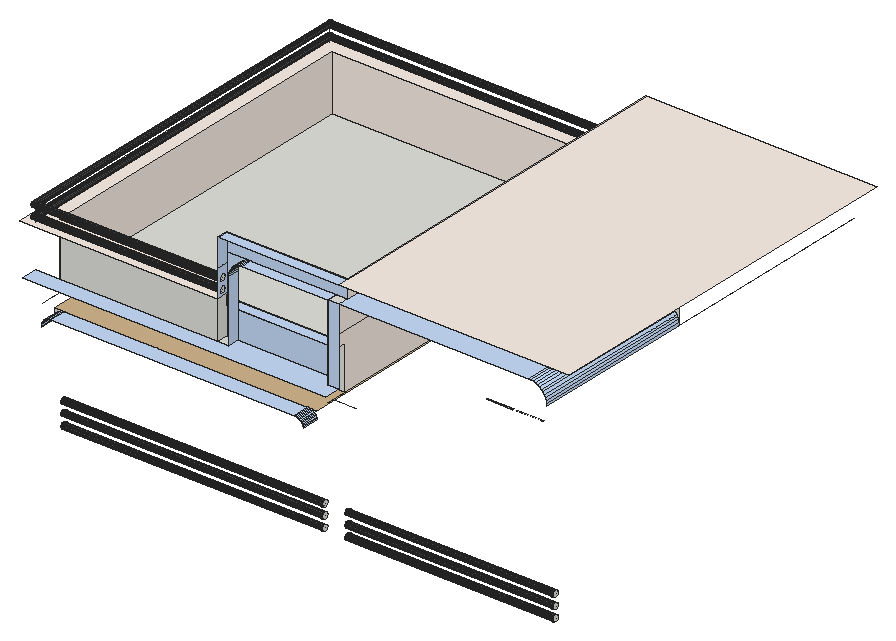
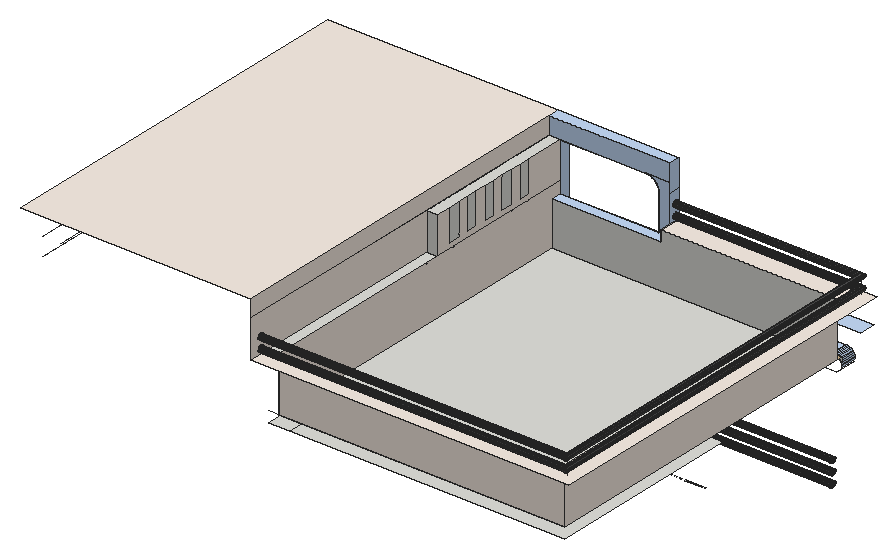
# SketchUp Ruby script. Lengths in inches.
U = 1.inch
M = Sketchup.active_model
def pt(a) = Geom::Point3d.new(a.map { |v| v * U })
def face(e, loops, mat)
  f = e.add_face(loops[0].map { |a| pt(a) })
  loops[1..].each { |l| e.add_face(l.map { |a| pt(a) }).erase! }
  f.material = f.back_material = mat if mat
  f
end
# faces: each face lists its corners as indices into pts; further lists are holes
def faces(e, pts, list, mat = nil) = list.each { |f| face(e, (f[0].is_a?(Array) ? f : [f]).map { |l| l.map { |i| pts[i] } }, mat) }
# xy, xz, yz: faces in a plane at the given z, y or x. An outline is a flat list of corners, or four numbers for a rectangle; further outlines are holes
def ring(l) = l.size == 4 ? [[l[0], l[1]], [l[2], l[1]], [l[2], l[3]], [l[0], l[3]]] : l.each_slice(2).to_a
def flat(e, list, mat, &to3) = list.each { |f| face(e, (f[0].is_a?(Array) ? f : [f]).map { |l| ring(l).map { |u, v| to3.(u, v) } }, mat) }
def xy(e, z, list, mat = nil) = flat(e, list, mat) { |x, y| [x, y, z] }
def xz(e, y, list, mat = nil) = flat(e, list, mat) { |x, z| [x, y, z] }
def yz(e, x, list, mat = nil) = flat(e, list, mat) { |y, z| [x, y, z] }
def lines(e, pts, list) = list.each { |a, b| e.add_line(pt(pts[a]), pt(pts[b])) }
# prism: a flat outline (further loops are holes) pulled along v
def prism(e, loops, v, mat = nil)
  f = face(e, loops, mat); d = Geom::Vector3d.new(v.map { |x| x * U })
  f.pushpull(f.normal.samedirection?(d) ? d.length : -d.length)
end
def box(e, o, s, mat = nil) = prism(e, [[o, [o[0] + s[0], o[1], o[2]], [o[0] + s[0], o[1] + s[1], o[2]], [o[0], o[1] + s[1], o[2]]]], [0, 0, s[2]], mat)
def at(x, y, z, deg = 0) = Geom::Transformation.translation(pt([x, y, z])) * Geom::Transformation.rotation(ORIGIN, Z_AXIS, deg.degrees)
def axes(o, x, y, z) = Geom::Transformation.new([*x, 0, *y, 0, *z, 0, *pt(o).to_a, 1])
def part(name) = M.definitions.add(name)
# library, detail: a bought-in or finely detailed component or shape, given as its bounding box
def library(name, o, s) = part(name).tap { |d| box(d.entities, o, s) }
def detail(e, o, s) = box(e.add_group.entities, o, s)
def put(e, d, t, mat = nil) = e.add_instance(d, t).tap { |i| i.material = mat if mat }
def group(e, t, mat = nil) = e.add_group.tap { |g| g.transformation = t; g.material = mat if mat }.entities
root = M.entities
M.materials.add("[0009_Linen]").color = [250, 240, 230]
M.materials.add("[0033_NavajoWhite]").color = [209, 182, 141]
M.materials.add("[0099_LightSteelBlue]").color = [198, 220, 249]
M.materials.add("[Metal Steel Textured White]").color = [84, 84, 84]
xy(root,427.88,[[43.43,263,65.05,264],[69.05,263,90.68,264],[366.6875,263,395.75,264],[399.75,263,428.8125,264]])
xy(root,428.88,[[148.81,264,198.81,266],[218.18,264,268.18,266]])
xy(root,480,[[114.29,108.66,111.1875,109.11,108.31,110.36,105.85,112.3,103.99,114.82,102.83,117.73,102.47,120.84,102.93,123.9375,104.17,126.8125,106.11,129.27,108.63,131.14,111.54,132.29,114.65,132.65,117.75,132.2,120.63,130.95,123.08,129.01,124.95,126.5,126.11,123.58,126.47,120.47,126.01,117.37,124.77,114.5,122.82,112.04,120.31,110.17,117.4,109.02],[234.29,108.66,231.1875,109.11,228.31,110.36,225.85,112.3,223.99,114.82,222.83,117.73,222.47,120.84,222.93,123.9375,224.17,126.8125,226.11,129.27,228.63,131.14,231.54,132.29,234.65,132.65,237.75,132.2,240.63,130.95,243.08,129.01,244.95,126.5,246.11,123.58,246.47,120.47,246.01,117.37,244.77,114.5,242.82,112.04,240.31,110.17,237.4,109.02],[24,264,324,480],[324,264,348,480]])
xy(root,480,[[[37.43,84,324,264],[114.29,108.66,117.4,109.02,120.31,110.17,122.82,112.04,124.77,114.5,126.01,117.37,126.47,120.47,126.11,123.58,124.95,126.5,123.08,129.01,120.63,130.95,117.75,132.2,114.65,132.65,111.54,132.29,108.63,131.14,106.11,129.27,104.17,126.8125,102.93,123.9375,102.47,120.84,102.83,117.73,103.99,114.82,105.85,112.3,108.31,110.36,111.1875,109.11],[234.29,108.66,237.4,109.02,240.31,110.17,242.82,112.04,244.77,114.5,246.01,117.37,246.47,120.47,246.11,123.58,244.95,126.5,243.08,129.01,240.63,130.95,237.75,132.2,234.65,132.65,231.54,132.29,228.63,131.14,226.11,129.27,224.17,126.8125,222.93,123.9375,222.47,120.84,222.83,117.73,223.99,114.82,225.85,112.3,228.31,110.36,231.1875,109.11]]],"[0033_NavajoWhite]")
xy(root,480,[[48.16,66,314.66,84]],"[0099_LightSteelBlue]")
xy(root,492,[[24,108,336,480]])
xy(root,510,[[216,84,228,96]])
xy(root,510,[[17.11,66,348,66,348,84,336,84,336,96,228,96,228,84,17.11,84]],"[0099_LightSteelBlue]")
xy(root,540,[[216,96,336,108]],"[0099_LightSteelBlue]")
xy(root,552,[[336,264,348,480]])
xy(root,552,[[0,84,216,84,216,108,24,108,24,480,348,480,348,504,0,504]],"[0009_Linen]")
xy(root,582,[[215.9375,84,216,96]])
xy(root,592.85,[[336,84,348,96],[336,96,348,264],[442.72,124.07,439.67,124.77,436.9,126.23,434.6,128.36,432.93,131.01,432.01,134.01,431.89,137.14,432.59,140.19,434.05,142.96,436.18,145.26,438.83,146.93,441.83,147.85,444.96,147.97,448.01,147.27,450.78,145.81,453.08,143.68,454.75,141.03,455.67,138.03,455.79,134.9,455.09,131.85,453.63,129.08,451.5,126.78,448.85,125.11,445.85,124.19]])
xy(root,592.85,[[242.86,84,336,96],[[348,84,556.05,264],[442.72,124.07,445.85,124.19,448.85,125.11,451.5,126.78,453.63,129.08,455.09,131.85,455.79,134.9,455.67,138.03,454.75,141.03,453.08,143.68,450.78,145.81,448.01,147.27,444.96,147.97,441.83,147.85,438.83,146.93,436.18,145.26,434.05,142.96,432.59,140.19,431.89,137.14,432.01,134.01,432.93,131.01,434.6,128.36,436.9,126.23,439.67,124.77]]],"[0099_LightSteelBlue]")
xy(root,612,[[348,84,600,504]],"[0009_Linen]")
xy(root,612,[[216,84,348,96]],"[0099_LightSteelBlue]")
xz(root,84,[[37.43,469.26,37.43,480,48.16,480,46.76,479.91,45.38,479.63,44.05,479.18,42.79,478.5625,41.625,477.78,40.57,476.85,39.64,475.8,38.86,474.63,38.24,473.37,37.79,472.04,37.52,470.66],[215.9375,582,216,592.85]])
xz(root,84,[[336,510,348,592.85]],"[0099_LightSteelBlue]")
xz(root,96,[[216,510,228,540],[215.9375,582,216,592.85]])
xz(root,96,[[228,510,336,540],[216,540,216,592.85,242.86,592.85,240.92,592.72,239.01,592.35,237.17,591.72,235.43,590.86,233.8125,589.78,232.35,588.5,231.07,587.04,229.99,585.42,229.13,583.68,228.51,581.84,228.13,579.93,228,577.99,228,540],[216,592.85,348,612]],"[0099_LightSteelBlue]")
xz(root,108,[[24,492,24,552,216,552,216,540,336,540,336,492]])
xz(root,264,[[336,552,348,592.85],[576,572.9,576,592.85,556.05,592.85,558.65,592.68,561.21,592.17,563.68,591.33,566.02,590.18,568.19,588.73,570.16,587.01,571.875,585.05,573.33,582.875,574.48,580.53,575.32,578.0625,575.83,575.5]])
xz(root,480,[[24,492,336,552]],"[0009_Linen]")
yz(root,24,[[108,492,480,552]],"[0009_Linen]")
yz(root,216,[[84,510,96,552],[96,540,108,552],[90,555,90.78,555.1,91.5,555.4,92.12,555.88,92.6,556.5,92.9,557.22,93,558,92.9,558.78,92.6,559.5,92.12,560.12,91.5,560.6,90.78,560.9,90,561,89.22,560.9,88.5,560.6,87.88,560.12,87.4,559.5,87.1,558.78,87,558,87.1,557.22,87.4,556.5,87.88,555.88,88.5,555.4,89.22,555.1],[90,567,90.78,567.1,91.5,567.4,92.12,567.88,92.6,568.5,92.9,569.22,93,570,92.9,570.78,92.6,571.5,92.12,572.12,91.5,572.6,90.78,572.9,90,573,89.22,572.9,88.5,572.6,87.88,572.12,87.4,571.5,87.1,570.78,87,570,87.1,569.22,87.4,568.5,87.88,567.88,88.5,567.4,89.22,567.1]])
yz(root,216,[[[84,552,96,582],[90,567,90.78,567.1,91.5,567.4,92.12,567.88,92.6,568.5,92.9,569.22,93,570,92.9,570.78,92.6,571.5,92.12,572.12,91.5,572.6,90.78,572.9,90,573,89.22,572.9,88.5,572.6,87.88,572.12,87.4,571.5,87.1,570.78,87,570,87.1,569.22,87.4,568.5,87.88,567.88,88.5,567.4,89.22,567.1],[90,555,90.78,555.1,91.5,555.4,92.12,555.88,92.6,556.5,92.9,557.22,93,558,92.9,558.78,92.6,559.5,92.12,560.12,91.5,560.6,90.78,560.9,90,561,89.22,560.9,88.5,560.6,87.88,560.12,87.4,559.5,87.1,558.78,87,558,87.1,557.22,87.4,556.5,87.88,555.88,88.5,555.4,89.22,555.1]],[84,582,96,612]],"[0099_LightSteelBlue]")
yz(root,228,[[84,510,96,577.99]],"[0099_LightSteelBlue]")
yz(root,324,[[96,357,96.78,357.1,97.5,357.4,98.12,357.88,98.6,358.5,98.9,359.22,99,360,98.9,360.78,98.6,361.5,98.12,362.12,97.5,362.6,96.78,362.9,96,363,95.22,362.9,94.5,362.6,93.88,362.12,93.4,361.5,93.1,360.78,93,360,93.1,359.22,93.4,358.5,93.88,357.88,94.5,357.4,95.22,357.1],[96,369,96.78,369.1,97.5,369.4,98.12,369.88,98.6,370.5,98.9,371.22,99,372,98.9,372.78,98.6,373.5,98.12,374.12,97.5,374.6,96.78,374.9,96,375,95.22,374.9,94.5,374.6,93.88,374.12,93.4,373.5,93.1,372.78,93,372,93.1,371.22,93.4,370.5,93.88,369.88,94.5,369.4,95.22,369.1],[96,381,96.78,381.1,97.5,381.4,98.12,381.88,98.6,382.5,98.9,383.22,99,384,98.9,384.78,98.6,385.5,98.12,386.12,97.5,386.6,96.78,386.9,96,387,95.22,386.9,94.5,386.6,93.88,386.12,93.4,385.5,93.1,384.78,93,384,93.1,383.22,93.4,382.5,93.88,381.88,94.5,381.4,95.22,381.1]])
yz(root,336,[[139.26,558.48,151.57,592.85],[163.26,558.48,175.57,592.85],[187.26,558.48,199.57,592.85],[211.26,558.48,223.57,592.85],[235.26,558.48,247.57,592.85]])
yz(root,336,[[108,492,108,540,96,540,96,552,480,552,480,492],[96,552,96,592.85,139.26,592.85,139.26,558.48,151.57,558.48,151.57,592.85,163.26,592.85,163.26,558.48,175.57,558.48,175.57,592.85,187.26,592.85,187.26,558.48,199.57,558.48,199.57,592.85,211.26,592.85,211.26,558.48,223.57,558.48,223.57,592.85,235.26,592.85,235.26,558.48,247.57,558.48,247.57,592.85,264,592.85,264,552]],"[0009_Linen]")
yz(root,336,[[84,510,96,592.85]],"[0099_LightSteelBlue]")
yz(root,348,[[[264,552,504,592.85],[492,567,492.78,567.1,493.5,567.4,494.12,567.88,494.6,568.5,494.9,569.22,495,570,494.9,570.78,494.6,571.5,494.12,572.12,493.5,572.6,492.78,572.9,492,573,491.22,572.9,490.5,572.6,489.88,572.12,489.4,571.5,489.1,570.78,489,570,489.1,569.22,489.4,568.5,489.88,567.88,490.5,567.4,491.22,567.1],[492,555,492.78,555.1,493.5,555.4,494.12,555.88,494.6,556.5,494.9,557.22,495,558,494.9,558.78,494.6,559.5,494.12,560.12,493.5,560.6,492.78,560.9,492,561,491.22,560.9,490.5,560.6,489.88,560.12,489.4,559.5,489.1,558.78,489,558,489.1,557.22,489.4,556.5,489.88,555.88,490.5,555.4,491.22,555.1]],[96,592.85,504,612]],"[0009_Linen]")
yz(root,576,[[96,357,96.78,357.1,97.5,357.4,98.12,357.88,98.6,358.5,98.9,359.22,99,360,98.9,360.78,98.6,361.5,98.12,362.12,97.5,362.6,96.78,362.9,96,363,95.22,362.9,94.5,362.6,93.88,362.12,93.4,361.5,93.1,360.78,93,360,93.1,359.22,93.4,358.5,93.88,357.88,94.5,357.4,95.22,357.1],[96,369,96.78,369.1,97.5,369.4,98.12,369.88,98.6,370.5,98.9,371.22,99,372,98.9,372.78,98.6,373.5,98.12,374.12,97.5,374.6,96.78,374.9,96,375,95.22,374.9,94.5,374.6,93.88,374.12,93.4,373.5,93.1,372.78,93,372,93.1,371.22,93.4,370.5,93.88,369.88,94.5,369.4,95.22,369.1],[96,381,96.78,381.1,97.5,381.4,98.12,381.88,98.6,382.5,98.9,383.22,99,384,98.9,384.78,98.6,385.5,98.12,386.12,97.5,386.6,96.78,386.9,96,387,95.22,386.9,94.5,386.6,93.88,386.12,93.4,385.5,93.1,384.78,93,384,93.1,383.22,93.4,382.5,93.88,381.88,94.5,381.4,95.22,381.1]])
p = [[324,96,357],[324,95.22,357.1],[37.43,95.22,357.1],[37.43,96,357],[576,96,357],[576,95.22,357.1],
  [348,95.22,357.1],[348,96,357],[324,96.78,357.1],[37.43,96.78,357.1],[576,96.78,357.1],[348,96.78,357.1],
  [324,94.5,357.4],[37.43,94.5,357.4],[576,94.5,357.4],[348,94.5,357.4],[324,97.5,357.4],[37.43,97.5,357.4],
  [576,97.5,357.4],[348,97.5,357.4],[324,93.88,357.88],[37.43,93.88,357.88],[576,93.88,357.88],[348,93.88,357.88],
  [324,98.12,357.88],[37.43,98.12,357.88],[576,98.12,357.88],[348,98.12,357.88],[324,93.4,358.5],[37.43,93.4,358.5],
  [576,93.4,358.5],[348,93.4,358.5],[324,98.6,358.5],[37.43,98.6,358.5],[576,98.6,358.5],[348,98.6,358.5],
  [324,93.1,359.22],[37.43,93.1,359.22],[576,93.1,359.22],[348,93.1,359.22],[324,98.9,359.22],[37.43,98.9,359.22],
  [576,98.9,359.22],[348,98.9,359.22],[324,93,360],[37.43,93,360],[576,93,360],[348,93,360],
  [324,99,360],[37.43,99,360],[576,99,360],[348,99,360],[324,93.1,360.78],[37.43,93.1,360.78],
  [576,93.1,360.78],[348,93.1,360.78],[324,98.9,360.78],[37.43,98.9,360.78],[576,98.9,360.78],[348,98.9,360.78],
  [324,93.4,361.5],[37.43,93.4,361.5],[576,93.4,361.5],[348,93.4,361.5],[324,98.6,361.5],[37.43,98.6,361.5],
  [576,98.6,361.5],[348,98.6,361.5],[324,93.88,362.12],[37.43,93.88,362.12],[576,93.88,362.12],[348,93.88,362.12],
  [324,98.12,362.12],[37.43,98.12,362.12],[576,98.12,362.12],[348,98.12,362.12],[324,94.5,362.6],[37.43,94.5,362.6],
  [576,94.5,362.6],[348,94.5,362.6],[324,97.5,362.6],[37.43,97.5,362.6],[576,97.5,362.6],[348,97.5,362.6],
  [324,95.22,362.9],[37.43,95.22,362.9],[576,95.22,362.9],[348,95.22,362.9],[324,96.78,362.9],[37.43,96.78,362.9],
  [576,96.78,362.9],[348,96.78,362.9],[324,96,363],[37.43,96,363],[576,96,363],[348,96,363],
  [324,96,369],[324,95.22,369.1],[37.43,95.22,369.1],[37.43,96,369],[576,96,369],[576,95.22,369.1],
  [348,95.22,369.1],[348,96,369],[324,96.78,369.1],[37.43,96.78,369.1],[576,96.78,369.1],[348,96.78,369.1],
  [324,94.5,369.4],[37.43,94.5,369.4],[576,94.5,369.4],[348,94.5,369.4],[324,97.5,369.4],[37.43,97.5,369.4],
  [576,97.5,369.4],[348,97.5,369.4],[324,93.88,369.88],[37.43,93.88,369.88],[576,93.88,369.88],[348,93.88,369.88],
  [324,98.12,369.88],[37.43,98.12,369.88],[576,98.12,369.88],[348,98.12,369.88],[324,93.4,370.5],[37.43,93.4,370.5],
  [576,93.4,370.5],[348,93.4,370.5],[324,98.6,370.5],[37.43,98.6,370.5],[576,98.6,370.5],[348,98.6,370.5],
  [324,93.1,371.22],[37.43,93.1,371.22],[576,93.1,371.22],[348,93.1,371.22],[324,98.9,371.22],[37.43,98.9,371.22],
  [576,98.9,371.22],[348,98.9,371.22],[324,93,372],[37.43,93,372],[576,93,372],[348,93,372],
  [324,99,372],[37.43,99,372],[576,99,372],[348,99,372],[324,93.1,372.78],[37.43,93.1,372.78],
  [576,93.1,372.78],[348,93.1,372.78],[324,98.9,372.78],[37.43,98.9,372.78],[576,98.9,372.78],[348,98.9,372.78],
  [324,93.4,373.5],[37.43,93.4,373.5],[576,93.4,373.5],[348,93.4,373.5],[324,98.6,373.5],[37.43,98.6,373.5],
  [576,98.6,373.5],[348,98.6,373.5],[324,93.88,374.12],[37.43,93.88,374.12],[576,93.88,374.12],[348,93.88,374.12],
  [324,98.12,374.12],[37.43,98.12,374.12],[576,98.12,374.12],[348,98.12,374.12],[324,94.5,374.6],[37.43,94.5,374.6],
  [576,94.5,374.6],[348,94.5,374.6],[324,97.5,374.6],[37.43,97.5,374.6],[576,97.5,374.6],[348,97.5,374.6],
  [324,95.22,374.9],[37.43,95.22,374.9],[576,95.22,374.9],[348,95.22,374.9],[324,96.78,374.9],[37.43,96.78,374.9],
  [576,96.78,374.9],[348,96.78,374.9],[324,96,375],[37.43,96,375],[576,96,375],[348,96,375],
  [324,96,381],[324,95.22,381.1],[37.43,95.22,381.1],[37.43,96,381],[576,96,381],[576,95.22,381.1],
  [348,95.22,381.1],[348,96,381],[324,96.78,381.1],[37.43,96.78,381.1],[576,96.78,381.1],[348,96.78,381.1],
  [324,94.5,381.4],[37.43,94.5,381.4],[576,94.5,381.4],[348,94.5,381.4],[324,97.5,381.4],[37.43,97.5,381.4],
  [576,97.5,381.4],[348,97.5,381.4],[324,93.88,381.88],[37.43,93.88,381.88],[576,93.88,381.88],[348,93.88,381.88],
  [324,98.12,381.88],[37.43,98.12,381.88],[576,98.12,381.88],[348,98.12,381.88],[324,93.4,382.5],[37.43,93.4,382.5],
  [576,93.4,382.5],[348,93.4,382.5],[324,98.6,382.5],[37.43,98.6,382.5],[576,98.6,382.5],[348,98.6,382.5],
  [324,93.1,383.22],[37.43,93.1,383.22],[576,93.1,383.22],[348,93.1,383.22],[324,98.9,383.22],[37.43,98.9,383.22],
  [576,98.9,383.22],[348,98.9,383.22],[324,93,384],[37.43,93,384],[576,93,384],[348,93,384],
  [324,99,384],[37.43,99,384],[576,99,384],[348,99,384],[324,93.1,384.78],[37.43,93.1,384.78],
  [576,93.1,384.78],[348,93.1,384.78],[324,98.9,384.78],[37.43,98.9,384.78],[576,98.9,384.78],[348,98.9,384.78],
  [324,93.4,385.5],[37.43,93.4,385.5],[576,93.4,385.5],[348,93.4,385.5],[324,98.6,385.5],[37.43,98.6,385.5],
  [576,98.6,385.5],[348,98.6,385.5],[324,93.88,386.12],[37.43,93.88,386.12],[576,93.88,386.12],[348,93.88,386.12],
  [324,98.12,386.12],[37.43,98.12,386.12],[576,98.12,386.12],[348,98.12,386.12],[324,94.5,386.6],[37.43,94.5,386.6],
  [576,94.5,386.6],[348,94.5,386.6],[324,97.5,386.6],[37.43,97.5,386.6],[576,97.5,386.6],[348,97.5,386.6],
  [324,95.22,386.9],[37.43,95.22,386.9],[576,95.22,386.9],[348,95.22,386.9],[324,96.78,386.9],[37.43,96.78,386.9],
  [576,96.78,386.9],[348,96.78,386.9],[324,96,387],[37.43,96,387],[576,96,387],[348,96,387],
  [37.43,84,469.26],[37.52,84,470.66],[37.52,66,470.66],[37.43,66,469.26],[37.79,84,472.04],[37.79,66,472.04],
  [323.92,84,471.88],[324,84,470.66],[324,66,470.66],[323.92,66,471.88],[323.68,84,473.08],[323.68,66,473.08],
  [38.24,84,473.37],[38.24,66,473.37],[323.29,84,474.24],[323.29,66,474.24],[38.86,84,474.63],[38.86,66,474.63],
  [322.75,84,475.33],[322.75,66,475.33],[39.64,84,475.8],[39.64,66,475.8],[322.07,84,476.35],[322.07,66,476.35],
  [40.57,84,476.85],[40.57,66,476.85],[321.27,84,477.27],[321.27,66,477.27],[41.625,84,477.78],[41.625,66,477.78],
  [320.35,84,478.07],[320.35,66,478.07],[42.79,84,478.5625],[42.79,66,478.5625],[319.33,84,478.75],[319.33,66,478.75],
  [44.05,84,479.18],[44.05,66,479.18],[318.24,84,479.29],[318.24,66,479.29],[45.38,84,479.63],[45.38,66,479.63],
  [317.08,84,479.68],[317.08,66,479.68],[46.76,84,479.91],[46.76,66,479.91],[315.88,84,479.92],[315.88,66,479.92],
  [48.16,84,480],[48.16,66,480],[314.66,84,480],[314.66,66,480],[216,90,555],[216,89.22,555.1],
  [11.22,89.22,555.1],[12,90,555],[11.22,492.78,555.1],[12,492,555],[216,90.78,555.1],[12.78,90.78,555.1],
  [12.78,491.22,555.1],[348,492,555],[348,491.22,555.1],[348,492.78,555.1],[216,88.5,555.4],[10.5,88.5,555.4],
  [10.5,493.5,555.4],[216,91.5,555.4],[13.5,91.5,555.4],[13.5,490.5,555.4],[348,490.5,555.4],[348,493.5,555.4],
  [216,87.88,555.88],[9.88,87.88,555.88],[9.88,494.12,555.88],[216,92.12,555.88],[14.12,92.12,555.88],[14.12,489.88,555.88],
  [348,489.88,555.88],[348,494.12,555.88],[216,87.4,556.5],[9.4,87.4,556.5],[9.4,494.6,556.5],[216,92.6,556.5],
  [14.6,92.6,556.5],[14.6,489.4,556.5],[348,489.4,556.5],[348,494.6,556.5],[216,87.1,557.22],[9.1,87.1,557.22],
  [9.1,494.9,557.22],[216,92.9,557.22],[14.9,92.9,557.22],[14.9,489.1,557.22],[348,489.1,557.22],[348,494.9,557.22],
  [216,87,558],[9,87,558],[9,495,558],[216,93,558],[15,93,558],[15,489,558],
  [348,489,558],[348,495,558],[216,87.1,558.78],[9.1,87.1,558.78],[9.1,494.9,558.78],[216,92.9,558.78],
  [14.9,92.9,558.78],[14.9,489.1,558.78],[348,489.1,558.78],[348,494.9,558.78],[216,87.4,559.5],[9.4,87.4,559.5],
  [9.4,494.6,559.5],[216,92.6,559.5],[14.6,92.6,559.5],[14.6,489.4,559.5],[348,489.4,559.5],[348,494.6,559.5],
  [216,87.88,560.12],[9.88,87.88,560.12],[9.88,494.12,560.12],[216,92.12,560.12],[14.12,92.12,560.12],[14.12,489.88,560.12],
  [348,489.88,560.12],[348,494.12,560.12],[216,88.5,560.6],[10.5,88.5,560.6],[10.5,493.5,560.6],[216,91.5,560.6],
  [13.5,91.5,560.6],[13.5,490.5,560.6],[348,490.5,560.6],[348,493.5,560.6],[216,89.22,560.9],[11.22,89.22,560.9],
  [11.22,492.78,560.9],[216,90.78,560.9],[12.78,90.78,560.9],[12.78,491.22,560.9],[348,491.22,560.9],[348,492.78,560.9],
  [216,90,561],[12,90,561],[12,492,561],[348,492,561],[216,90,567],[216,89.22,567.1],
  [11.22,89.22,567.1],[12,90,567],[11.22,492.78,567.1],[12,492,567],[216,90.78,567.1],[12.78,90.78,567.1],
  [12.78,491.22,567.1],[348,492,567],[348,491.22,567.1],[348,492.78,567.1],[216,88.5,567.4],[10.5,88.5,567.4],
  [10.5,493.5,567.4],[216,91.5,567.4],[13.5,91.5,567.4],[13.5,490.5,567.4],[348,490.5,567.4],[348,493.5,567.4],
  [216,87.88,567.88],[9.88,87.88,567.88],[9.88,494.12,567.88],[216,92.12,567.88],[14.12,92.12,567.88],[14.12,489.88,567.88],
  [348,489.88,567.88],[348,494.12,567.88],[216,87.4,568.5],[9.4,87.4,568.5],[9.4,494.6,568.5],[216,92.6,568.5],
  [14.6,92.6,568.5],[14.6,489.4,568.5],[348,489.4,568.5],[348,494.6,568.5],[216,87.1,569.22],[9.1,87.1,569.22],
  [9.1,494.9,569.22],[216,92.9,569.22],[14.9,92.9,569.22],[14.9,489.1,569.22],[348,489.1,569.22],[348,494.9,569.22],
  [216,87,570],[9,87,570],[9,495,570],[216,93,570],[15,93,570],[15,489,570],
  [348,489,570],[348,495,570],[216,87.1,570.78],[9.1,87.1,570.78],[9.1,494.9,570.78],[216,92.9,570.78],
  [14.9,92.9,570.78],[14.9,489.1,570.78],[348,489.1,570.78],[348,494.9,570.78],[216,87.4,571.5],[9.4,87.4,571.5],
  [9.4,494.6,571.5],[216,92.6,571.5],[14.6,92.6,571.5],[14.6,489.4,571.5],[348,489.4,571.5],[348,494.6,571.5],
  [216,87.88,572.12],[9.88,87.88,572.12],[9.88,494.12,572.12],[216,92.12,572.12],[14.12,92.12,572.12],[14.12,489.88,572.12],
  [348,489.88,572.12],[348,494.12,572.12],[216,88.5,572.6],[10.5,88.5,572.6],[10.5,493.5,572.6],[216,91.5,572.6],
  [13.5,91.5,572.6],[13.5,490.5,572.6],[348,490.5,572.6],[348,493.5,572.6],[216,89.22,572.9],[11.22,89.22,572.9],
  [11.22,492.78,572.9],[216,90.78,572.9],[12.78,90.78,572.9],[12.78,491.22,572.9],[348,491.22,572.9],[348,492.78,572.9],
  [575.83,84,575.5],[575.83,264,575.5],[576,264,572.9],[576,84,572.9],[216,90,573],[12,90,573],
  [12,492,573],[348,492,573],[575.32,84,578.0625],[575.32,264,578.0625],[228.13,84,579.93],[228,84,577.99],
  [228,96,577.99],[228.13,96,579.93],[574.48,84,580.53],[574.48,264,580.53],[228.51,84,581.84],[228.51,96,581.84],
  [573.33,84,582.875],[573.33,264,582.875],[229.13,84,583.68],[229.13,96,583.68],[571.875,84,585.05],[571.875,264,585.05],
  [229.99,84,585.42],[229.99,96,585.42],[570.16,84,587.01],[570.16,264,587.01],[231.07,84,587.04],[231.07,96,587.04],
  [232.35,84,588.5],[232.35,96,588.5],[568.19,84,588.73],[568.19,264,588.73],[233.8125,84,589.78],[233.8125,96,589.78],
  [566.02,84,590.18],[566.02,264,590.18],[235.43,84,590.86],[235.43,96,590.86],[563.68,84,591.33],[563.68,264,591.33],
  [237.17,84,591.72],[237.17,96,591.72],[561.21,84,592.17],[561.21,264,592.17],[239.01,84,592.35],[239.01,96,592.35],
  [558.65,84,592.68],[558.65,264,592.68],[240.92,84,592.72],[240.92,96,592.72],[242.86,84,592.85],[242.86,96,592.85],
  [556.05,84,592.85],[556.05,264,592.85],[324,108,480],[348,108,480],[336,108,492],[336,84,492],
  [336,480,492],[348,480,492],[336,480,549.9375],[348,480,549.9375],[24,108,480],[37.43,108,480],
  [24,84,480],[324,84,480],[324,66,480],[576,264,592.85],[576,504,592.85],[556.05,504,592.85],
  [576,504,572.9],[576,96,384],[348,96,384],[324,96,384],[37.43,96,384],[37.43,96,372],
  [324,96,372],[37.43,96,360],[324,96,360],[348,96,372],[576,96,372],[348,96,360],
  [576,96,360],[12,90,552],[12,90,570],[216,90,570],[12,492,570],[12,492,552],
  [348,492,570],[12,90,558],[216,90,558],[12,492,558],[348,492,558]]
faces(root,p,[[0,1,2,3],[4,5,6,7],[8,0,3,9],[10,4,7,11],[1,12,13,2],[5,14,15,6],[16,8,9,17],[18,10,11,19],
  [12,20,21,13],[14,22,23,15],[24,16,17,25],[26,18,19,27],[20,28,29,21],[22,30,31,23],[32,24,25,33],[34,26,27,35],
  [28,36,37,29],[30,38,39,31],[40,32,33,41],[42,34,35,43],[36,44,45,37],[38,46,47,39],[48,40,41,49],[50,42,43,51],
  [44,52,53,45],[46,54,55,47],[56,48,49,57],[58,50,51,59],[52,60,61,53],[54,62,63,55],[64,56,57,65],[66,58,59,67],
  [60,68,69,61],[62,70,71,63],[72,64,65,73],[74,66,67,75],[68,76,77,69],[70,78,79,71],[80,72,73,81],[82,74,75,83],
  [76,84,85,77],[78,86,87,79],[88,80,81,89],[90,82,83,91],[84,92,93,85],[86,94,95,87],[92,88,89,93],[94,90,91,95],
  [96,97,98,99],[100,101,102,103],[104,96,99,105],[106,100,103,107],[97,108,109,98],[101,110,111,102],[112,104,105,113],[114,106,107,115],
  [108,116,117,109],[110,118,119,111],[120,112,113,121],[122,114,115,123],[116,124,125,117],[118,126,127,119],[128,120,121,129],[130,122,123,131],
  [124,132,133,125],[126,134,135,127],[136,128,129,137],[138,130,131,139],[132,140,141,133],[134,142,143,135],[144,136,137,145],[146,138,139,147],
  [140,148,149,141],[142,150,151,143],[152,144,145,153],[154,146,147,155],[148,156,157,149],[150,158,159,151],[160,152,153,161],[162,154,155,163],
  [156,164,165,157],[158,166,167,159],[168,160,161,169],[170,162,163,171],[164,172,173,165],[166,174,175,167],[176,168,169,177],[178,170,171,179],
  [172,180,181,173],[174,182,183,175],[184,176,177,185],[186,178,179,187],[180,188,189,181],[182,190,191,183],[188,184,185,189],[190,186,187,191],
  [192,193,194,195],[196,197,198,199],[200,192,195,201],[202,196,199,203],[193,204,205,194],[197,206,207,198],[208,200,201,209],[210,202,203,211],
  [204,212,213,205],[206,214,215,207],[216,208,209,217],[218,210,211,219],[212,220,221,213],[214,222,223,215],[224,216,217,225],[226,218,219,227],
  [220,228,229,221],[222,230,231,223],[232,224,225,233],[234,226,227,235],[228,236,237,229],[230,238,239,231],[240,232,233,241],[242,234,235,243],
  [236,244,245,237],[238,246,247,239],[248,240,241,249],[250,242,243,251],[244,252,253,245],[246,254,255,247],[256,248,249,257],[258,250,251,259],
  [252,260,261,253],[254,262,263,255],[264,256,257,265],[266,258,259,267],[260,268,269,261],[262,270,271,263],[272,264,265,273],[274,266,267,275],
  [268,276,277,269],[270,278,279,271],[280,272,273,281],[282,274,275,283],[276,284,285,277],[278,286,287,279],[284,280,281,285],[286,282,283,287],
  [340,341,342,343],[343,342,344,345],[346,340,343,347],[347,343,345,348],[348,345,349,350],[345,344,351,349],[341,352,353,342],[342,353,354,344],
  [355,346,347,356],[356,347,348,357],[357,348,350,358],[344,354,359,351],[352,360,361,353],[353,361,362,354],[363,355,356,364],[364,356,357,365],
  [365,357,358,366],[354,362,367,359],[360,368,369,361],[361,369,370,362],[371,363,364,372],[372,364,365,373],[373,365,366,374],[362,370,375,367],
  [368,376,377,369],[369,377,378,370],[379,371,372,380],[380,372,373,381],[381,373,374,382],[370,378,383,375],[376,384,385,377],[377,385,386,378],
  [387,379,380,388],[388,380,381,389],[389,381,382,390],[378,386,391,383],[384,392,393,385],[385,393,394,386],[395,387,388,396],[396,388,389,397],
  [397,389,390,398],[386,394,399,391],[392,400,401,393],[393,401,402,394],[403,395,396,404],[404,396,397,405],[405,397,398,406],[394,402,407,399],
  [400,408,409,401],[401,409,410,402],[411,403,404,412],[412,404,405,413],[413,405,406,414],[402,410,415,407],[408,416,417,409],[409,417,418,410],
  [419,411,412,420],[420,412,413,421],[421,413,414,422],[410,418,423,415],[416,424,425,417],[417,425,426,418],[427,419,420,428],[428,420,421,429],
  [429,421,422,430],[418,426,431,423],[424,432,433,425],[425,433,434,426],[432,427,428,433],[433,428,429,434],[434,429,430,435],[426,434,435,431],
  [436,437,438,439],[439,438,440,441],[442,436,439,443],[443,439,441,444],[444,441,445,446],[441,440,447,445],[437,448,449,438],[438,449,450,440],
  [451,442,443,452],[452,443,444,453],[453,444,446,454],[440,450,455,447],[448,456,457,449],[449,457,458,450],[459,451,452,460],[460,452,453,461],
  [461,453,454,462],[450,458,463,455],[456,464,465,457],[457,465,466,458],[467,459,460,468],[468,460,461,469],[469,461,462,470],[458,466,471,463],
  [464,472,473,465],[465,473,474,466],[475,467,468,476],[476,468,469,477],[477,469,470,478],[466,474,479,471],[472,480,481,473],[473,481,482,474],
  [483,475,476,484],[484,476,477,485],[485,477,478,486],[474,482,487,479],[480,488,489,481],[481,489,490,482],[491,483,484,492],[492,484,485,493],
  [493,485,486,494],[482,490,495,487],[488,496,497,489],[489,497,498,490],[499,491,492,500],[500,492,493,501],[501,493,494,502],[490,498,503,495],
  [496,504,505,497],[497,505,506,498],[507,499,500,508],[508,500,501,509],[509,501,502,510],[498,506,511,503],[504,512,513,505],[505,513,514,506],
  [515,507,508,516],[516,508,509,517],[517,509,510,518],[506,514,519,511],[512,520,521,513],[513,521,522,514],[523,515,516,524],[524,516,517,525],
  [525,517,518,526],[514,522,527,519],[520,532,533,521],[521,533,534,522],[532,523,524,533],[533,524,525,534],[534,525,526,535],[522,534,535,527]],"[Metal Steel Textured White]")
faces(root,p,[[288,289,290,291],[289,292,293,290],[294,295,296,297],[298,294,297,299],[292,300,301,293],[302,298,299,303],[300,304,305,301],[306,302,303,307],
  [304,308,309,305],[310,306,307,311],[308,312,313,309],[314,310,311,315],[312,316,317,313],[318,314,315,319],[316,320,321,317],[322,318,319,323],
  [320,324,325,321],[326,322,323,327],[324,328,329,325],[330,326,327,331],[328,332,333,329],[334,330,331,335],[332,336,337,333],[338,334,335,339],
  [528,529,530,531],[536,537,529,528],[538,539,540,541],[542,543,537,536],[544,538,541,545],[546,547,543,542],[548,544,545,549],[550,551,547,546],
  [552,548,549,553],[554,555,551,550],[556,552,553,557],[558,556,557,559],[560,561,555,554],[562,558,559,563],[564,565,561,560],[566,562,563,567],
  [568,569,565,564],[570,566,567,571],[572,573,569,568],[574,570,571,575],[576,577,573,572],[578,574,575,579],[580,578,579,581],[582,583,577,576]],"[0099_LightSteelBlue]")
lines(root,p,[[584,585],[586,587],[588,589],[590,591],[592,593],[592,594],[595,596],[597,598],[583,599],[530,600],[601,602],[602,199],
  [603,604],[604,195],[605,99],[606,605],[607,3],[608,607],[609,103],[610,609],[611,7],[612,611],[191,609],[95,611],
  [189,605],[93,607],[613,343],[614,615],[614,616],[617,345],[616,618],[619,433],[620,619],[621,434],[619,621],[621,622],
  [439,614],[441,616],[343,619],[345,621],[433,439],[434,441]])
